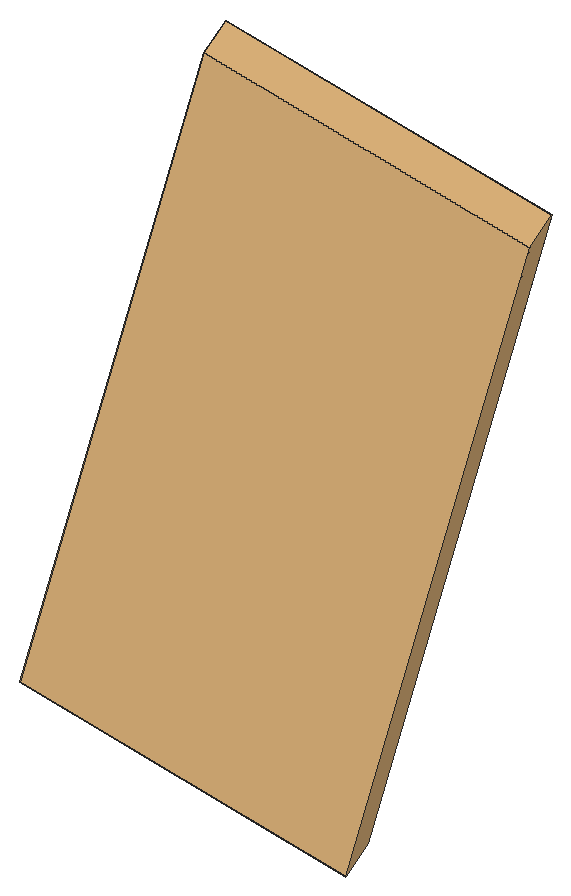
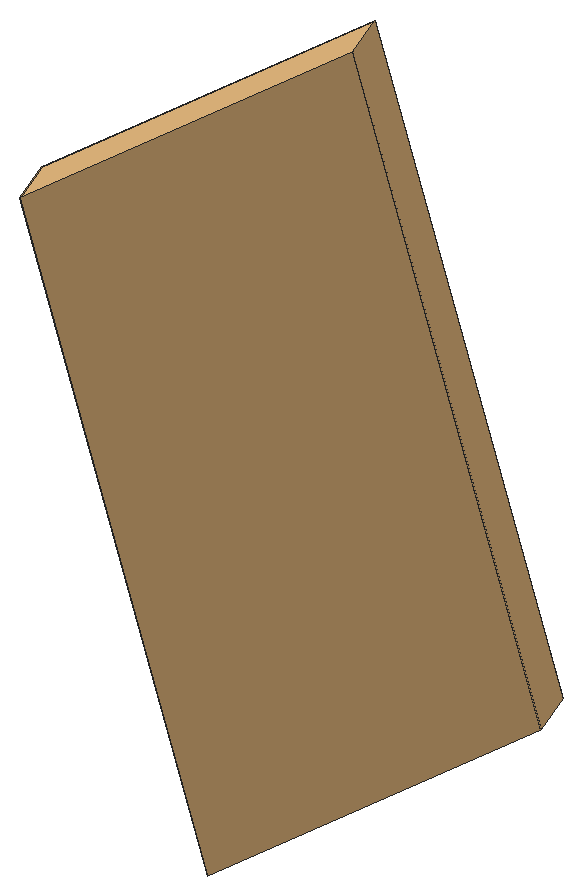
# SketchUp Ruby script. Lengths in inches.
U = 1.inch
M = Sketchup.active_model
def pt(a) = Geom::Point3d.new(a.map { |v| v * U })
def face(e, loops, mat)
  f = e.add_face(loops[0].map { |a| pt(a) })
  loops[1..].each { |l| e.add_face(l.map { |a| pt(a) }).erase! }
  f.material = f.back_material = mat if mat
  f
end
# faces: each face lists its corners as indices into pts; further lists are holes
def faces(e, pts, list, mat = nil) = list.each { |f| face(e, (f[0].is_a?(Array) ? f : [f]).map { |l| l.map { |i| pts[i] } }, mat) }
# xy, xz, yz: faces in a plane at the given z, y or x. An outline is a flat list of corners, or four numbers for a rectangle; further outlines are holes
def ring(l) = l.size == 4 ? [[l[0], l[1]], [l[2], l[1]], [l[2], l[3]], [l[0], l[3]]] : l.each_slice(2).to_a
def flat(e, list, mat, &to3) = list.each { |f| face(e, (f[0].is_a?(Array) ? f : [f]).map { |l| ring(l).map { |u, v| to3.(u, v) } }, mat) }
def xy(e, z, list, mat = nil) = flat(e, list, mat) { |x, y| [x, y, z] }
def xz(e, y, list, mat = nil) = flat(e, list, mat) { |x, z| [x, y, z] }
def yz(e, x, list, mat = nil) = flat(e, list, mat) { |y, z| [x, y, z] }
def lines(e, pts, list) = list.each { |a, b| e.add_line(pt(pts[a]), pt(pts[b])) }
# prism: a flat outline (further loops are holes) pulled along v
def prism(e, loops, v, mat = nil)
  f = face(e, loops, mat); d = Geom::Vector3d.new(v.map { |x| x * U })
  f.pushpull(f.normal.samedirection?(d) ? d.length : -d.length)
end
def box(e, o, s, mat = nil) = prism(e, [[o, [o[0] + s[0], o[1], o[2]], [o[0] + s[0], o[1] + s[1], o[2]], [o[0], o[1] + s[1], o[2]]]], [0, 0, s[2]], mat)
def at(x, y, z, deg = 0) = Geom::Transformation.translation(pt([x, y, z])) * Geom::Transformation.rotation(ORIGIN, Z_AXIS, deg.degrees)
def axes(o, x, y, z) = Geom::Transformation.new([*x, 0, *y, 0, *z, 0, *pt(o).to_a, 1])
def part(name) = M.definitions.add(name)
# library, detail: a bought-in or finely detailed component or shape, given as its bounding box
def library(name, o, s) = part(name).tap { |d| box(d.entities, o, s) }
def detail(e, o, s) = box(e.add_group.entities, o, s)
def put(e, d, t, mat = nil) = e.add_instance(d, t).tap { |i| i.material = mat if mat }
def group(e, t, mat = nil) = e.add_group.tap { |g| g.transformation = t; g.material = mat if mat }.entities
root = M.entities
c1 = library("sm2 st v2 Component\#1",[0,0,0],[29.46,4.93,43.46])
put(root,c1,axes([81.5,102.7,34.53],[-0.34978,-0.19812,0.23587],[0.16968,-0.46612,-0.00617],[0.13657,0.07168,0.61177]))
